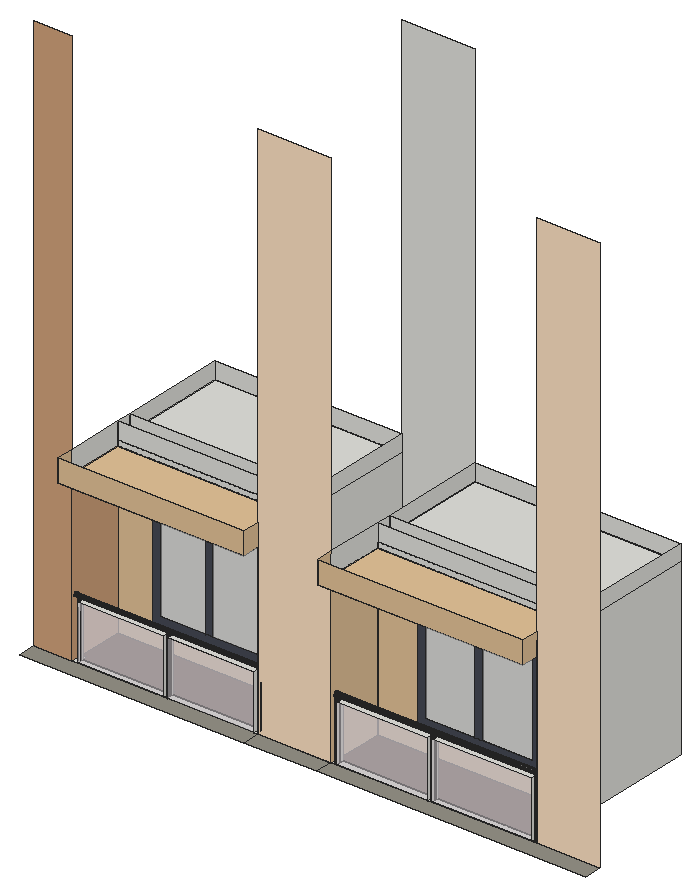
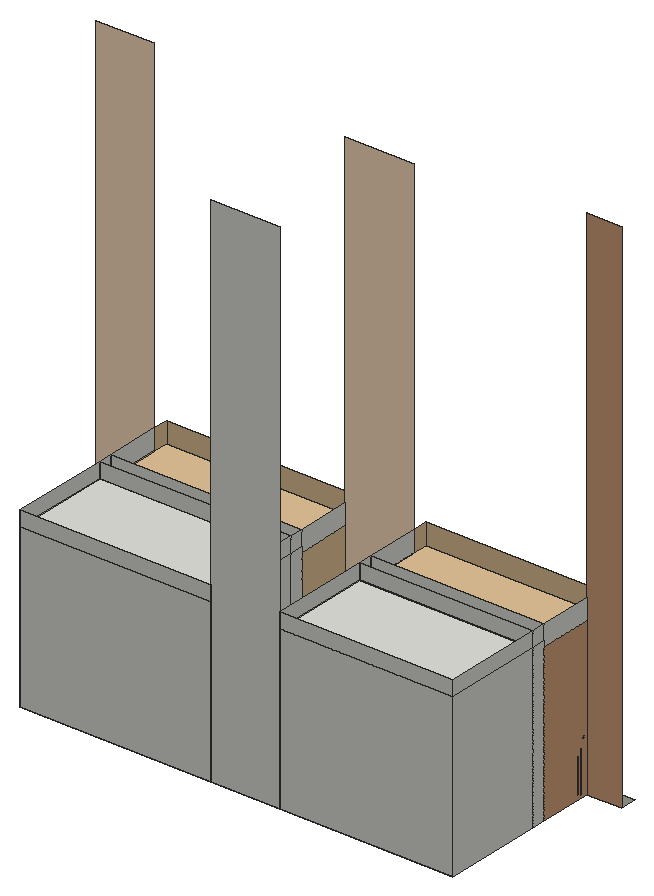
# SketchUp Ruby script. Lengths in inches.
U = 1.inch
M = Sketchup.active_model
def pt(a) = Geom::Point3d.new(a.map { |v| v * U })
def face(e, loops, mat)
  f = e.add_face(loops[0].map { |a| pt(a) })
  loops[1..].each { |l| e.add_face(l.map { |a| pt(a) }).erase! }
  f.material = f.back_material = mat if mat
  f
end
# faces: each face lists its corners as indices into pts; further lists are holes
def faces(e, pts, list, mat = nil) = list.each { |f| face(e, (f[0].is_a?(Array) ? f : [f]).map { |l| l.map { |i| pts[i] } }, mat) }
# xy, xz, yz: faces in a plane at the given z, y or x. An outline is a flat list of corners, or four numbers for a rectangle; further outlines are holes
def ring(l) = l.size == 4 ? [[l[0], l[1]], [l[2], l[1]], [l[2], l[3]], [l[0], l[3]]] : l.each_slice(2).to_a
def flat(e, list, mat, &to3) = list.each { |f| face(e, (f[0].is_a?(Array) ? f : [f]).map { |l| ring(l).map { |u, v| to3.(u, v) } }, mat) }
def xy(e, z, list, mat = nil) = flat(e, list, mat) { |x, y| [x, y, z] }
def xz(e, y, list, mat = nil) = flat(e, list, mat) { |x, z| [x, y, z] }
def yz(e, x, list, mat = nil) = flat(e, list, mat) { |y, z| [x, y, z] }
def lines(e, pts, list) = list.each { |a, b| e.add_line(pt(pts[a]), pt(pts[b])) }
# prism: a flat outline (further loops are holes) pulled along v
def prism(e, loops, v, mat = nil)
  f = face(e, loops, mat); d = Geom::Vector3d.new(v.map { |x| x * U })
  f.pushpull(f.normal.samedirection?(d) ? d.length : -d.length)
end
def box(e, o, s, mat = nil) = prism(e, [[o, [o[0] + s[0], o[1], o[2]], [o[0] + s[0], o[1] + s[1], o[2]], [o[0], o[1] + s[1], o[2]]]], [0, 0, s[2]], mat)
def at(x, y, z, deg = 0) = Geom::Transformation.translation(pt([x, y, z])) * Geom::Transformation.rotation(ORIGIN, Z_AXIS, deg.degrees)
def axes(o, x, y, z) = Geom::Transformation.new([*x, 0, *y, 0, *z, 0, *pt(o).to_a, 1])
def part(name) = M.definitions.add(name)
# library, detail: a bought-in or finely detailed component or shape, given as its bounding box
def library(name, o, s) = part(name).tap { |d| box(d.entities, o, s) }
def detail(e, o, s) = box(e.add_group.entities, o, s)
def put(e, d, t, mat = nil) = e.add_instance(d, t).tap { |i| i.material = mat if mat }
def group(e, t, mat = nil) = e.add_group.tap { |g| g.transformation = t; g.material = mat if mat }.entities
root = M.entities
M.materials.add("[0035_Tan]").color = [229, 196, 153]
M.materials.add("[Cladding Siding Tan]").color = [211, 164, 124]
M.materials.add("[Color M05]").color = [114, 114, 114]
M.materials.add("[Formica Graystone]").color = [149, 146, 135]
M.materials.add("[Formica Laminate Dark]").color = [70, 74, 84]
M.materials.add("[Formica Laminate Light]").color = [255, 226, 196]
M.materials.add("[Suede Brown]").color = [61, 41, 32]
M.materials.add("[Translucent Glass Gray]").color = [214, 214, 214]
M.materials["[Translucent Glass Gray]"].alpha = 0.5
M.materials.add("[Translucent Glass Safety]1").color = [244, 237, 242]
M.materials["[Translucent Glass Safety]1"].alpha = 0.5
xy(root,285.1875,[[[225.05,423.82,232.5,438.71],[230.48,427.9,230.08,427.95,229.7,428.11,229.38,428.36,229.13,428.68,228.97,429.06,228.92,429.46,228.97,429.86,229.13,430.24,229.38,430.56,229.7,430.8125,230.08,430.97,230.48,431.02,230.89,430.97,231.26,430.8125,231.59,430.56,231.84,430.24,231.99,429.86,232.04,429.46,231.99,429.06,231.84,428.68,231.59,428.36,231.26,428.11,230.89,427.95]],[232.5,423.82,341.97,433.08],[[341.97,423.82,345.48,438.71],[343.73,427.9,343.33,427.95,342.95,428.11,342.63,428.36,342.38,428.68,342.22,429.06,342.17,429.46,342.22,429.86,342.38,430.24,342.63,430.56,342.95,430.8125,343.33,430.97,343.73,431.02,344.14,430.97,344.51,430.8125,344.84,430.56,345.09,430.24,345.24,429.86,345.29,429.46,345.24,429.06,345.09,428.68,344.84,428.36,344.51,428.11,344.14,427.95]],[345.48,423.82,456.12,433.08],[[456.12,423.82,460.75,438.71],[457.79,427.9,457.39,427.95,457.01,428.11,456.69,428.36,456.44,428.68,456.29,429.06,456.23,429.46,456.29,429.86,456.44,430.24,456.69,430.56,457.01,430.8125,457.39,430.97,457.79,431.02,458.2,430.97,458.58,430.8125,458.9,430.56,459.15,430.24,459.3,429.86,459.36,429.46,459.3,429.06,459.15,428.68,458.9,428.36,458.58,428.11,458.2,427.95]],
  [460.75,423.82,553.875,651.39],[[553.875,423.82,560.86,434.81],[558.14,426.4,557.5,426.48,556.89,426.73,556.375,427.13,555.98,427.65,555.73,428.25,555.64,428.9,555.73,429.54,555.98,430.15,556.375,430.66,556.89,431.0625,557.5,431.31,558.14,431.4,558.79,431.31,559.39,431.0625,559.91,430.66,560.31,430.15,560.56,429.54,560.64,428.9,560.56,428.25,560.31,427.65,559.91,427.13,559.39,426.73,558.79,426.48]],[560.86,423.82,675.79,432.75],[[675.79,423.82,681.35,434.81],[678.52,426.4,677.87,426.48,677.27,426.73,676.75,427.13,676.35,427.65,676.1,428.25,676.02,428.9,676.1,429.54,676.35,430.15,676.75,430.66,677.27,431.0625,677.87,431.31,678.52,431.4,679.17,431.31,679.77,431.0625,680.29,430.66,680.68,430.15,680.93,429.54,681.02,428.9,680.93,428.25,680.68,427.65,680.29,427.13,679.77,426.73,679.17,426.48]],[681.35,423.82,807.3,432.75],
  [[807.3,423.82,814,434.81],[810.08,426.4,809.43,426.48,808.83,426.73,808.3125,427.13,807.92,427.65,807.67,428.25,807.58,428.9,807.67,429.54,807.92,430.15,808.3125,430.66,808.83,431.0625,809.43,431.31,810.08,431.4,810.73,431.31,811.33,431.0625,811.85,430.66,812.25,430.15,812.5,429.54,812.58,428.9,812.5,428.25,812.25,427.65,811.85,427.13,811.33,426.73,810.73,426.48]],[558.14,426.4,557.5,426.48,556.89,426.73,556.375,427.13,555.98,427.65,555.73,428.25,555.64,428.9,555.73,429.54,555.98,430.15,556.375,430.66,556.89,431.0625,557.5,431.31,558.14,431.4,558.79,431.31,559.39,431.0625,559.91,430.66,560.31,430.15,560.56,429.54,560.64,428.9,560.56,428.25,560.31,427.65,559.91,427.13,559.39,426.73,558.79,426.48],[678.52,426.4,677.87,426.48,677.27,426.73,676.75,427.13,676.35,427.65,676.1,428.25,676.02,428.9,676.1,429.54,676.35,430.15,676.75,430.66,677.27,431.0625,677.87,431.31,678.52,431.4,679.17,431.31,679.77,431.0625,680.29,430.66,680.68,430.15,680.93,429.54,681.02,428.9,680.93,428.25,680.68,427.65,680.29,427.13,679.77,426.73,679.17,426.48],[810.08,426.4,809.43,426.48,808.83,426.73,808.3125,427.13,807.92,427.65,807.67,428.25,807.58,428.9,807.67,429.54,807.92,430.15,808.3125,430.66,808.83,431.0625,809.43,431.31,810.08,431.4,810.73,431.31,811.33,431.0625,811.85,430.66,812.25,430.15,812.5,429.54,812.58,428.9,812.5,428.25,812.25,427.65,811.85,427.13,811.33,426.73,810.73,426.48],[230.48,427.9,230.08,427.95,229.7,428.11,229.38,428.36,229.13,428.68,228.97,429.06,228.92,429.46,228.97,429.86,229.13,430.24,229.38,430.56,229.7,430.8125,230.08,430.97,230.48,431.02,230.89,430.97,231.26,430.8125,231.59,430.56,231.84,430.24,231.99,429.86,232.04,429.46,231.99,429.06,231.84,428.68,231.59,428.36,231.26,428.11,230.89,427.95],
  [343.73,427.9,343.33,427.95,342.95,428.11,342.63,428.36,342.38,428.68,342.22,429.06,342.17,429.46,342.22,429.86,342.38,430.24,342.63,430.56,342.95,430.8125,343.33,430.97,343.73,431.02,344.14,430.97,344.51,430.8125,344.84,430.56,345.09,430.24,345.24,429.86,345.29,429.46,345.24,429.06,345.09,428.68,344.84,428.36,344.51,428.11,344.14,427.95],[457.79,427.9,457.39,427.95,457.01,428.11,456.69,428.36,456.44,428.68,456.29,429.06,456.23,429.46,456.29,429.86,456.44,430.24,456.69,430.56,457.01,430.8125,457.39,430.97,457.79,431.02,458.2,430.97,458.58,430.8125,458.9,430.56,459.15,430.24,459.3,429.86,459.36,429.46,459.3,429.06,459.15,428.68,458.9,428.36,458.58,428.11,458.2,427.95],[225.05,496.86,460.75,515.85],[553.875,496.86,814,515.85],[225.05,515.85,460.75,651.39],
  [553.875,515.85,814,651.39]])
xy(root,285.1875,[[177.7,401.69,460.75,423.82],[460.75,401.69,553.875,423.82],[553.875,401.69,893.35,423.82]],"[Formica Graystone]")
xy(root,285.1875,[[560.86,432.75,675.79,432.75,675.79,434.81,681.35,434.81,681.35,432.75,807.3,432.75,807.3,434.81,814,434.81,814,496.86,553.875,496.86,553.875,434.81,560.86,434.81],[232.5,433.08,341.97,433.08,341.97,438.71,345.48,438.71,345.48,433.08,456.12,433.08,456.12,438.71,460.75,438.71,460.75,496.86,225.05,496.86,225.05,438.71,232.5,438.71]],"[Suede Brown]")
xy(root,354.1875,[[232.5,423.82,341.97,433.08],[345.48,423.82,456.12,433.08]])
xy(root,356.625,[[560.86,423.82,675.79,432.75],[681.35,423.82,807.3,432.75]])
xy(root,358.5,[[343.73,427.9,344.14,427.95,344.51,428.11,344.84,428.36,345.09,428.68,345.24,429.06,345.29,429.46,345.24,429.86,345.09,430.24,344.84,430.56,344.51,430.8125,344.14,430.97,343.73,431.02,343.33,430.97,342.95,430.8125,342.63,430.56,342.38,430.24,342.22,429.86,342.17,429.46,342.22,429.06,342.38,428.68,342.63,428.36,342.95,428.11,343.33,427.95]])
xy(root,359.125,[[457.79,427.9,458.2,427.95,458.58,428.11,458.9,428.36,459.15,428.68,459.3,429.06,459.36,429.46,459.3,429.86,459.15,430.24,458.9,430.56,458.58,430.8125,458.2,430.97,457.79,431.02,457.39,430.97,457.01,430.8125,456.69,430.56,456.44,430.24,456.29,429.86,456.23,429.46,456.29,429.06,456.44,428.68,456.69,428.36,457.01,428.11,457.39,427.95]])
xy(root,359.35,[[230.48,427.9,230.89,427.95,231.26,428.11,231.59,428.36,231.84,428.68,231.99,429.06,232.04,429.46,231.99,429.86,231.84,430.24,231.59,430.56,231.26,430.8125,231.07,430.89,229.9,430.89,229.7,430.8125,229.38,430.56,229.13,430.24,228.97,429.86,228.92,429.46,228.97,429.06,229.13,428.68,229.38,428.36,229.7,428.11,230.08,427.95],[229.9,430.89,231.07,430.89,230.89,430.97,230.48,431.02,230.08,430.97]])
xy(root,360.5,[[810.08,426.4,810.73,426.48,811.33,426.73,811.85,427.13,812.25,427.65,812.5,428.25,812.58,428.9,812.5,429.54,812.25,430.15,811.85,430.66,811.33,431.0625,810.73,431.31,810.08,431.4,809.43,431.31,808.83,431.0625,808.3125,430.66,807.92,430.15,807.67,429.54,807.58,428.9,807.67,428.25,807.92,427.65,808.3125,427.13,808.83,426.73,809.43,426.48]])
xy(root,360.8125,[[678.52,426.4,679.17,426.48,679.77,426.73,680.29,427.13,680.68,427.65,680.93,428.25,681.02,428.9,680.93,429.54,680.68,430.15,680.29,430.66,679.77,431.0625,679.17,431.31,678.52,431.4,677.87,431.31,677.27,431.0625,676.75,430.66,676.35,430.15,676.1,429.54,676.02,428.9,676.1,428.25,676.35,427.65,676.75,427.13,677.27,426.73,677.87,426.48]])
xy(root,361.35,[[558.14,426.4,558.79,426.48,559.39,426.73,559.86,427.09,556.43,427.09,556.89,426.73,557.5,426.48],[556.43,427.09,559.86,427.09,559.91,427.13,560.31,427.65,560.56,428.25,560.64,428.9,560.56,429.54,560.31,430.15,559.91,430.66,559.39,431.0625,558.79,431.31,558.14,431.4,557.5,431.31,556.89,431.0625,556.375,430.66,555.98,430.15,555.73,429.54,555.64,428.9,555.73,428.25,555.98,427.65,556.375,427.13]])
xy(root,496.625,[[225.05,402.38,460.75,496.86],[553.875,402.38,814,496.86]],"[0035_Tan]")
xy(root,504,[[225.05,496.86,460.75,515.85],[553.875,496.86,814,515.85],[225.05,515.85,460.75,651.39],[553.875,515.85,814,651.39]])
xz(root,402.38,[[225.05,496.625,460.75,524.8125],[553.875,496.625,814,524.8125]],"[0035_Tan]")
xz(root,423.82,[[345.48,285.1875,346.91,354.1875]])
xz(root,423.82,[[177.7,285.1875,225.05,994.25]],"[Cladding Siding Tan]")
xz(root,423.82,[[460.75,285.1875,553.875,971.5],[814,285.1875,893.35,994.25]],"[Formica Laminate Light]")
xz(root,423.82,[[232.5,285.1875,341.97,354.1875],[346.91,285.1875,456.12,354.1875],[560.86,285.1875,675.79,356.625],[681.35,285.1875,807.3,356.625]],"[Translucent Glass Safety]1")
xz(root,432.75,[[560.86,285.1875,675.79,356.625],[681.35,285.1875,807.3,356.625]],"[Translucent Glass Safety]1")
xz(root,433.08,[[232.5,285.1875,341.97,354.1875],[345.48,285.1875,456.12,354.1875]],"[Translucent Glass Safety]1")
xz(root,496.86,[[225.05,496.625,460.75,504],[553.875,496.625,814,504],[225.05,504,460.75,524.8125],[553.875,504,814,524.8125]])
xz(root,496.86,[[[225.05,285.1875,460.75,496.625],[269.29,311.6875,412.47,477.3125]],[[553.875,285.1875,814,496.625],[604.28,313.48,762.28,471.48]]],"[0035_Tan]")
xz(root,496.86,[[[269.29,311.6875,412.47,477.3125],[279.54,321.95,402.22,467.06]],[[604.28,313.48,762.28,471.48],[615.53,324.73,751.03,460.23]],[336.36,321.95,346,467.06],[676.75,324.73,687.68,460.23]],"[Formica Laminate Dark]")
xz(root,496.86,[[279.54,321.95,336.36,467.06],[346,321.95,402.22,467.06],[615.53,324.73,676.75,460.23],[687.68,324.73,751.03,460.23]],"[Translucent Glass Gray]")
xz(root,515.85,[[225.05,285.1875,460.75,504],[553.875,285.1875,814,504],[225.05,504,460.75,524.8125],[553.875,504,814,524.8125]])
xz(root,651.39,[[225.05,285.1875,460.75,504],[460.75,285.1875,553.875,994.25],[553.875,285.1875,814,504],[225.05,504,460.75,524.8125],[553.875,504,814,524.8125]])
yz(root,225.05,[[496.86,285.1875,515.85,504],[515.85,285.1875,651.39,504],[428.9,356.75,428.37,356.82,427.87,357.03,427.44,357.36,427.12,357.78,426.91,358.28,426.84,358.8125,426.91,359.35,427.12,359.85,427.44,360.27,427.87,360.6,428.37,360.81,428.9,360.875,429.4375,360.81,429.93,360.6,430.36,360.27,430.6875,359.85,430.89,359.35,430.96,358.8125,430.89,358.28,430.6875,357.78,430.36,357.36,429.93,357.03,429.4375,356.82],[423.82,496.625,496.86,524.8125],[496.86,504,515.85,524.8125],
  [515.85,504,651.39,524.8125]])
yz(root,225.05,[[402.38,496.625,423.82,524.8125]],"[0035_Tan]")
yz(root,225.05,[[[423.82,285.1875,496.86,496.625],[428.9,356.75,428.37,356.82,427.87,357.03,427.44,357.36,427.12,357.78,426.91,358.28,426.84,358.8125,426.91,359.35,427.12,359.85,427.44,360.27,427.87,360.6,428.37,360.81,428.9,360.875,429.4375,360.81,429.93,360.6,430.36,360.27,430.6875,359.85,430.89,359.35,430.96,358.8125,430.89,358.28,430.6875,357.78,430.36,357.36,429.93,357.03,429.4375,356.82]]],"[Cladding Siding Tan]")
yz(root,232.5,[[423.82,285.1875,433.08,354.1875]])
yz(root,341.97,[[423.82,285.1875,433.08,354.1875]])
yz(root,345.48,[[423.82,285.1875,433.08,354.1875]])
yz(root,456.12,[[423.82,285.1875,433.08,354.1875]])
yz(root,460.75,[[496.86,285.1875,515.85,504],[515.85,285.1875,651.39,504],[423.82,496.625,496.86,524.8125],[496.86,504,515.85,524.8125],[515.85,504,651.39,524.8125]])
yz(root,460.75,[[[423.82,285.1875,496.86,496.625],[428.9,356.75,429.4375,356.82,429.93,357.03,430.36,357.36,430.6875,357.78,430.89,358.28,430.96,358.8125,430.89,359.35,430.6875,359.85,430.36,360.27,429.93,360.6,429.4375,360.81,428.9,360.875,428.37,360.81,427.87,360.6,427.44,360.27,427.12,359.85,426.91,359.35,426.84,358.8125,426.91,358.28,427.12,357.78,427.44,357.36,427.87,357.03,428.37,356.82]],[402.38,496.625,423.82,524.8125]],"[0035_Tan]")
yz(root,553.875,[[496.86,285.1875,515.85,504],[515.85,285.1875,651.39,504],[429.78,358.66,429.08,358.75,428.43,359.02,427.875,359.45,427.45,360,427.18,360.65,427.09,361.35,427.18,362.04,427.45,362.69,427.875,363.25,428.43,363.67,429.08,363.94,429.78,364.03,430.47,363.94,431.12,363.67,431.68,363.25,432.1,362.69,432.37,362.04,432.46,361.35,432.37,360.65,432.1,360,431.68,359.45,431.12,359.02,430.47,358.75],[423.82,496.625,496.86,524.8125],[496.86,504,515.85,524.8125],
  [515.85,504,651.39,524.8125]])
yz(root,553.875,[[[423.82,285.1875,496.86,496.625],[429.78,358.66,429.08,358.75,428.43,359.02,427.875,359.45,427.45,360,427.18,360.65,427.09,361.35,427.18,362.04,427.45,362.69,427.875,363.25,428.43,363.67,429.08,363.94,429.78,364.03,430.47,363.94,431.12,363.67,431.68,363.25,432.1,362.69,432.37,362.04,432.46,361.35,432.37,360.65,432.1,360,431.68,359.45,431.12,359.02,430.47,358.75]],[402.38,496.625,423.82,524.8125]],"[0035_Tan]")
yz(root,560.86,[[423.82,285.1875,432.75,356.625]])
yz(root,675.79,[[423.82,285.1875,432.75,356.625]])
yz(root,681.35,[[423.82,285.1875,432.75,356.625]])
yz(root,807.3,[[423.82,285.1875,432.75,356.625]])
yz(root,814,[[496.86,285.1875,515.85,504],[515.85,285.1875,651.39,504],[423.82,496.625,496.86,524.8125],[496.86,504,515.85,524.8125],[515.85,504,651.39,524.8125]])
yz(root,814,[[[423.82,285.1875,496.86,496.625],[429.78,358.66,430.47,358.75,431.12,359.02,431.68,359.45,432.1,360,432.37,360.65,432.46,361.35,432.37,362.04,432.1,362.69,431.68,363.25,431.12,363.67,430.47,363.94,429.78,364.03,429.08,363.94,428.43,363.67,427.875,363.25,427.45,362.69,427.18,362.04,427.09,361.35,427.18,360.65,427.45,360,427.875,359.45,428.43,359.02,429.08,358.75]],[402.38,496.625,423.82,524.8125]],"[0035_Tan]")
p = [[557.5,426.48,285.1875],[558.14,426.4,285.1875],[558.14,426.4,361.35],[557.5,426.48,361.35],[558.79,426.48,285.1875],[558.79,426.48,361.35],
  [677.87,426.48,285.1875],[678.52,426.4,285.1875],[678.52,426.4,360.8125],[677.87,426.48,360.8125],[679.17,426.48,285.1875],[679.17,426.48,360.8125],
  [809.43,426.48,285.1875],[810.08,426.4,285.1875],[810.08,426.4,360.5],[809.43,426.48,360.5],[810.73,426.48,285.1875],[810.73,426.48,360.5],
  [556.89,426.73,285.1875],[556.89,426.73,361.35],[559.39,426.73,285.1875],[559.39,426.73,361.35],[677.27,426.73,285.1875],[677.27,426.73,360.8125],
  [679.77,426.73,285.1875],[679.77,426.73,360.8125],[808.83,426.73,285.1875],[808.83,426.73,360.5],[811.33,426.73,285.1875],[811.33,426.73,360.5],
  [556.375,427.13,285.1875],[556.43,427.09,361.35],[556.375,427.13,361.35],[559.91,427.13,285.1875],[559.91,427.13,361.35],[559.86,427.09,361.35],
  [676.75,427.13,285.1875],[676.75,427.13,360.8125],[680.29,427.13,285.1875],[680.29,427.13,360.8125],[808.3125,427.13,285.1875],[808.3125,427.13,360.5],
  [811.85,427.13,285.1875],[811.85,427.13,360.5],[555.98,427.65,285.1875],[555.98,427.65,361.35],[560.31,427.65,285.1875],[560.31,427.65,361.35],
  [676.35,427.65,285.1875],[676.35,427.65,360.8125],[680.68,427.65,285.1875],[680.68,427.65,360.8125],[807.92,427.65,285.1875],[807.92,427.65,360.5],
  [812.25,427.65,285.1875],[812.25,427.65,360.5],[555.73,428.25,285.1875],[555.73,428.25,361.35],[560.56,428.25,285.1875],[560.56,428.25,361.35],
  [676.1,428.25,285.1875],[676.1,428.25,360.8125],[680.93,428.25,285.1875],[680.93,428.25,360.8125],[807.67,428.25,285.1875],[807.67,428.25,360.5],
  [812.5,428.25,285.1875],[812.5,428.25,360.5],[230.08,427.95,285.1875],[230.48,427.9,285.1875],[230.48,427.9,359.35],[230.08,427.95,359.35],
  [230.89,427.95,285.1875],[230.89,427.95,359.35],[343.33,427.95,285.1875],[343.73,427.9,285.1875],[343.73,427.9,358.5],[343.33,427.95,358.5],
  [344.14,427.95,285.1875],[344.14,427.95,358.5],[457.39,427.95,285.1875],[457.79,427.9,285.1875],[457.79,427.9,359.125],[457.39,427.95,359.125],
  [458.2,427.95,285.1875],[458.2,427.95,359.125],[229.7,428.11,285.1875],[229.7,428.11,359.35],[231.26,428.11,285.1875],[231.26,428.11,359.35],
  [342.95,428.11,285.1875],[342.95,428.11,358.5],[344.51,428.11,285.1875],[344.51,428.11,358.5],[457.01,428.11,285.1875],[457.01,428.11,359.125],
  [458.58,428.11,285.1875],[458.58,428.11,359.125],[229.38,428.36,285.1875],[229.38,428.36,359.35],[231.59,428.36,285.1875],[231.59,428.36,359.35],
  [342.63,428.36,285.1875],[342.63,428.36,358.5],[344.84,428.36,285.1875],[344.84,428.36,358.5],[456.69,428.36,285.1875],[456.69,428.36,359.125],
  [458.9,428.36,285.1875],[458.9,428.36,359.125],[555.64,428.9,285.1875],[555.64,428.9,361.35],[560.64,428.9,285.1875],[560.64,428.9,361.35],
  [676.02,428.9,285.1875],[676.02,428.9,360.8125],[681.02,428.9,285.1875],[681.02,428.9,360.8125],[807.58,428.9,285.1875],[807.58,428.9,360.5],
  [812.58,428.9,285.1875],[812.58,428.9,360.5],[229.13,428.68,285.1875],[229.13,428.68,359.35],[231.84,428.68,285.1875],[231.84,428.68,359.35],
  [342.38,428.68,285.1875],[342.38,428.68,358.5],[345.09,428.68,285.1875],[345.09,428.68,358.5],[456.44,428.68,285.1875],[456.44,428.68,359.125],
  [459.15,428.68,285.1875],[459.15,428.68,359.125],[228.97,429.06,285.1875],[228.97,429.06,359.35],[231.99,429.06,285.1875],[231.99,429.06,359.35],
  [342.22,429.06,285.1875],[342.22,429.06,358.5],[345.24,429.06,285.1875],[345.24,429.06,358.5],[456.29,429.06,285.1875],[456.29,429.06,359.125],
  [459.3,429.06,285.1875],[459.3,429.06,359.125],[555.73,429.54,285.1875],[555.73,429.54,361.35],[560.56,429.54,285.1875],[560.56,429.54,361.35],
  [676.1,429.54,285.1875],[676.1,429.54,360.8125],[680.93,429.54,285.1875],[680.93,429.54,360.8125],[807.67,429.54,285.1875],[807.67,429.54,360.5],
  [812.5,429.54,285.1875],[812.5,429.54,360.5],[228.92,429.46,285.1875],[228.92,429.46,359.35],[232.04,429.46,285.1875],[232.04,429.46,359.35],
  [342.17,429.46,285.1875],[342.17,429.46,358.5],[345.29,429.46,285.1875],[345.29,429.46,358.5],[456.23,429.46,285.1875],[456.23,429.46,359.125],
  [459.36,429.46,285.1875],[459.36,429.46,359.125],[228.97,429.86,285.1875],[228.97,429.86,359.35],[231.99,429.86,285.1875],[231.99,429.86,359.35],
  [342.22,429.86,285.1875],[342.22,429.86,358.5],[345.24,429.86,285.1875],[345.24,429.86,358.5],[456.29,429.86,285.1875],[456.29,429.86,359.125],
  [459.3,429.86,285.1875],[459.3,429.86,359.125],[555.98,430.15,285.1875],[555.98,430.15,361.35],[560.31,430.15,285.1875],[560.31,430.15,361.35],
  [676.35,430.15,285.1875],[676.35,430.15,360.8125],[680.68,430.15,285.1875],[680.68,430.15,360.8125],[807.92,430.15,285.1875],[807.92,430.15,360.5],
  [812.25,430.15,285.1875],[812.25,430.15,360.5],[229.13,430.24,285.1875],[229.13,430.24,359.35],[231.84,430.24,285.1875],[231.84,430.24,359.35],
  [342.38,430.24,285.1875],[342.38,430.24,358.5],[345.09,430.24,285.1875],[345.09,430.24,358.5],[456.44,430.24,285.1875],[456.44,430.24,359.125],
  [459.15,430.24,285.1875],[459.15,430.24,359.125],[556.375,430.66,285.1875],[556.375,430.66,361.35],[559.91,430.66,285.1875],[559.91,430.66,361.35],
  [676.75,430.66,285.1875],[676.75,430.66,360.8125],[680.29,430.66,285.1875],[680.29,430.66,360.8125],[808.3125,430.66,285.1875],[808.3125,430.66,360.5],
  [811.85,430.66,285.1875],[811.85,430.66,360.5],[229.38,430.56,285.1875],[229.38,430.56,359.35],[231.59,430.56,285.1875],[231.59,430.56,359.35],
  [342.63,430.56,285.1875],[342.63,430.56,358.5],[344.84,430.56,285.1875],[344.84,430.56,358.5],[456.69,430.56,285.1875],[456.69,430.56,359.125],
  [458.9,430.56,285.1875],[458.9,430.56,359.125],[229.7,430.8125,285.1875],[229.7,430.8125,359.35],[231.26,430.8125,285.1875],[231.26,430.8125,359.35],
  [342.95,430.8125,285.1875],[342.95,430.8125,358.5],[344.51,430.8125,285.1875],[344.51,430.8125,358.5],[457.01,430.8125,285.1875],[457.01,430.8125,359.125],
  [458.58,430.8125,285.1875],[458.58,430.8125,359.125],[556.89,431.0625,285.1875],[556.89,431.0625,361.35],[559.39,431.0625,285.1875],[559.39,431.0625,361.35],
  [677.27,431.0625,285.1875],[677.27,431.0625,360.8125],[679.77,431.0625,285.1875],[679.77,431.0625,360.8125],[808.83,431.0625,285.1875],[808.83,431.0625,360.5],
  [811.33,431.0625,285.1875],[811.33,431.0625,360.5],[230.08,430.97,285.1875],[229.9,430.89,359.35],[230.08,430.97,359.35],[230.89,430.97,285.1875],
  [230.89,430.97,359.35],[231.07,430.89,359.35],[343.33,430.97,285.1875],[343.33,430.97,358.5],[344.14,430.97,285.1875],[344.14,430.97,358.5],
  [457.39,430.97,285.1875],[457.39,430.97,359.125],[458.2,430.97,285.1875],[458.2,430.97,359.125],[230.48,431.02,285.1875],[230.48,431.02,359.35],
  [343.73,431.02,285.1875],[343.73,431.02,358.5],[457.79,431.02,285.1875],[457.79,431.02,359.125],[557.5,431.31,285.1875],[557.5,431.31,361.35],
  [558.79,431.31,285.1875],[558.79,431.31,361.35],[677.87,431.31,285.1875],[677.87,431.31,360.8125],[679.17,431.31,285.1875],[679.17,431.31,360.8125],
  [809.43,431.31,285.1875],[809.43,431.31,360.5],[810.73,431.31,285.1875],[810.73,431.31,360.5],[558.14,431.4,285.1875],[558.14,431.4,361.35],
  [678.52,431.4,285.1875],[678.52,431.4,360.8125],[810.08,431.4,285.1875],[810.08,431.4,360.5],[225.05,427.87,357.03],[225.05,428.37,356.82],
  [460.75,428.37,356.82],[460.75,427.87,357.03],[225.05,428.9,356.75],[460.75,428.9,356.75],[225.05,429.4375,356.82],[460.75,429.4375,356.82],
  [225.05,429.93,357.03],[460.75,429.93,357.03],[225.05,427.44,357.36],[460.75,427.44,357.36],[225.05,430.36,357.36],[460.75,430.36,357.36],
  [225.05,427.12,357.78],[460.75,427.12,357.78],[225.05,430.6875,357.78],[460.75,430.6875,357.78],[225.05,426.91,358.28],[460.75,426.91,358.28],
  [225.05,430.89,358.28],[460.75,430.89,358.28],[225.05,426.84,358.8125],[460.75,426.84,358.8125],[225.05,430.96,358.8125],[460.75,430.96,358.8125],
  [553.875,429.08,358.75],[553.875,429.78,358.66],[814,429.78,358.66],[814,429.08,358.75],[553.875,430.47,358.75],[814,430.47,358.75],
  [225.05,426.91,359.35],[460.75,426.91,359.35],[553.875,428.43,359.02],[814,428.43,359.02],[553.875,431.12,359.02],[814,431.12,359.02],
  [225.05,430.89,359.35],[460.75,430.89,359.35],[553.875,427.875,359.45],[814,427.875,359.45],[553.875,431.68,359.45],[814,431.68,359.45],
  [225.05,427.12,359.85],[460.75,427.12,359.85],[225.05,430.6875,359.85],[460.75,430.6875,359.85],[553.875,427.45,360],[814,427.45,360],
  [553.875,432.1,360],[814,432.1,360],[225.05,427.44,360.27],[460.75,427.44,360.27],[225.05,430.36,360.27],[460.75,430.36,360.27],
  [553.875,427.18,360.65],[814,427.18,360.65],[553.875,432.37,360.65],[814,432.37,360.65],[225.05,427.87,360.6],[460.75,427.87,360.6],
  [225.05,429.93,360.6],[460.75,429.93,360.6],[225.05,428.37,360.81],[460.75,428.37,360.81],[225.05,429.4375,360.81],[460.75,429.4375,360.81],
  [553.875,427.09,361.35],[814,427.09,361.35],[553.875,432.46,361.35],[814,432.46,361.35],[225.05,428.9,360.875],[460.75,428.9,360.875],
  [553.875,427.18,362.04],[814,427.18,362.04],[553.875,432.37,362.04],[814,432.37,362.04],[553.875,427.45,362.69],[814,427.45,362.69],
  [553.875,432.1,362.69],[814,432.1,362.69],[553.875,427.875,363.25],[814,427.875,363.25],[553.875,431.68,363.25],[814,431.68,363.25],
  [553.875,428.43,363.67],[814,428.43,363.67],[553.875,431.12,363.67],[814,431.12,363.67],[553.875,429.08,363.94],[814,429.08,363.94],
  [553.875,430.47,363.94],[814,430.47,363.94],[553.875,429.78,364.03],[814,429.78,364.03]]
faces(root,p,[[0,1,2,3],[1,4,5,2],[6,7,8,9],[7,10,11,8],[12,13,14,15],[13,16,17,14],[18,0,3,19],[4,20,21,5],
  [22,6,9,23],[10,24,25,11],[26,12,15,27],[16,28,29,17],[30,18,19,31,32],[20,33,34,35,21],[36,22,23,37],[24,38,39,25],
  [40,26,27,41],[28,42,43,29],[44,30,32,45],[33,46,47,34],[48,36,37,49],[38,50,51,39],[52,40,41,53],[42,54,55,43],
  [56,44,45,57],[46,58,59,47],[60,48,49,61],[50,62,63,51],[64,52,53,65],[54,66,67,55],[68,69,70,71],[69,72,73,70],
  [74,75,76,77],[75,78,79,76],[80,81,82,83],[81,84,85,82],[86,68,71,87],[72,88,89,73],[90,74,77,91],[78,92,93,79],
  [94,80,83,95],[84,96,97,85],[98,86,87,99],[88,100,101,89],[102,90,91,103],[92,104,105,93],[106,94,95,107],[96,108,109,97],
  [110,56,57,111],[58,112,113,59],[114,60,61,115],[62,116,117,63],[118,64,65,119],[66,120,121,67],[122,98,99,123],[100,124,125,101],
  [126,102,103,127],[104,128,129,105],[130,106,107,131],[108,132,133,109],[134,122,123,135],[124,136,137,125],[138,126,127,139],[128,140,141,129],
  [142,130,131,143],[132,144,145,133],[146,110,111,147],[112,148,149,113],[150,114,115,151],[116,152,153,117],[154,118,119,155],[120,156,157,121],
  [158,134,135,159],[136,160,161,137],[162,138,139,163],[140,164,165,141],[166,142,143,167],[144,168,169,145],[170,158,159,171],[160,172,173,161],
  [174,162,163,175],[164,176,177,165],[178,166,167,179],[168,180,181,169],[182,146,147,183],[148,184,185,149],[186,150,151,187],[152,188,189,153],
  [190,154,155,191],[156,192,193,157],[194,170,171,195],[172,196,197,173],[198,174,175,199],[176,200,201,177],[202,178,179,203],[180,204,205,181],
  [206,182,183,207],[184,208,209,185],[210,186,187,211],[188,212,213,189],[214,190,191,215],[192,216,217,193],[218,194,195,219],[196,220,221,197],
  [222,198,199,223],[200,224,225,201],[226,202,203,227],[204,228,229,205],[230,218,219,231],[220,232,233,221],[234,222,223,235],[224,236,237,225],
  [238,226,227,239],[228,240,241,229],[242,206,207,243],[208,244,245,209],[246,210,211,247],[212,248,249,213],[250,214,215,251],[216,252,253,217],
  [254,230,231,255,256],[232,257,258,259,233],[260,234,235,261],[236,262,263,237],[264,238,239,265],[240,266,267,241],[268,254,256,269],[257,268,269,258],
  [270,260,261,271],[262,270,271,263],[272,264,265,273],[266,272,273,267],[274,242,243,275],[244,276,277,245],[278,246,247,279],[248,280,281,249],
  [282,250,251,283],[252,284,285,253],[286,274,275,287],[276,286,287,277],[288,278,279,289],[280,288,289,281],[290,282,283,291],[284,290,291,285],
  [292,293,294,295],[293,296,297,294],[296,298,299,297],[298,300,301,299],[302,292,295,303],[300,304,305,301],[306,302,303,307],[304,308,309,305],
  [310,306,307,311],[308,312,313,309],[314,310,311,315],[312,316,317,313],[318,319,320,321],[319,322,323,320],[324,314,315,325],[326,318,321,327],
  [322,328,329,323],[316,330,255,259,331,317],[332,326,327,333],[328,334,335,329],[336,324,325,337],[330,338,339,331,259,255],[340,332,333,341],[334,342,343,335],
  [344,336,337,345],[338,346,347,339],[348,340,341,349],[342,350,351,343],[352,344,345,353],[346,354,355,347],[356,352,353,357],[354,358,359,355],
  [360,348,349,361,35,31],[350,362,363,351],[364,356,357,365],[358,364,365,359],[366,360,31,35,361,367],[362,368,369,363],[370,366,367,371],[368,372,373,369],
  [374,370,371,375],[372,376,377,373],[378,374,375,379],[376,380,381,377],[382,378,379,383],[380,384,385,381],[386,382,383,387],[384,386,387,385]],"[Color M05]")
